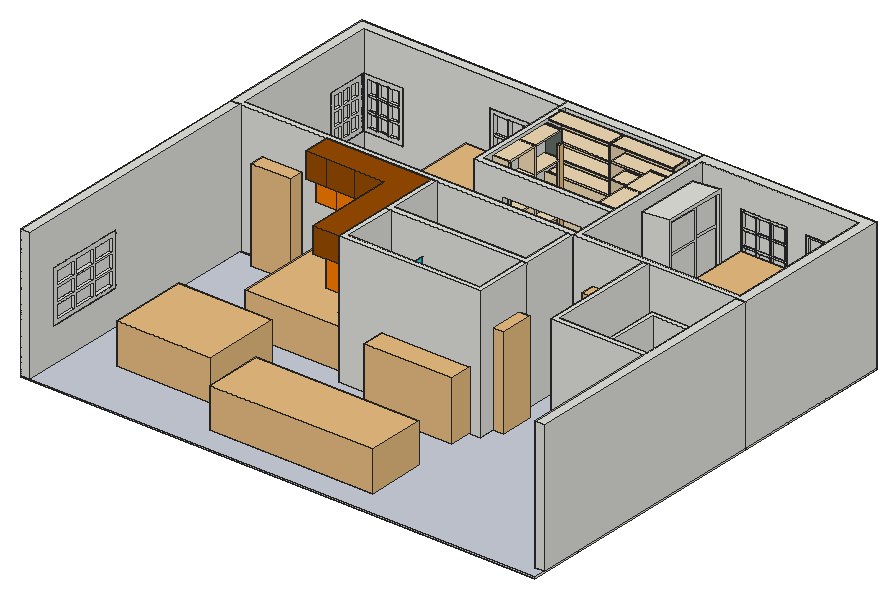
# SketchUp Ruby script. Lengths in inches.
U = 1.inch
M = Sketchup.active_model
def pt(a) = Geom::Point3d.new(a.map { |v| v * U })
def face(e, loops, mat)
  f = e.add_face(loops[0].map { |a| pt(a) })
  loops[1..].each { |l| e.add_face(l.map { |a| pt(a) }).erase! }
  f.material = f.back_material = mat if mat
  f
end
# faces: each face lists its corners as indices into pts; further lists are holes
def faces(e, pts, list, mat = nil) = list.each { |f| face(e, (f[0].is_a?(Array) ? f : [f]).map { |l| l.map { |i| pts[i] } }, mat) }
# xy, xz, yz: faces in a plane at the given z, y or x. An outline is a flat list of corners, or four numbers for a rectangle; further outlines are holes
def ring(l) = l.size == 4 ? [[l[0], l[1]], [l[2], l[1]], [l[2], l[3]], [l[0], l[3]]] : l.each_slice(2).to_a
def flat(e, list, mat, &to3) = list.each { |f| face(e, (f[0].is_a?(Array) ? f : [f]).map { |l| ring(l).map { |u, v| to3.(u, v) } }, mat) }
def xy(e, z, list, mat = nil) = flat(e, list, mat) { |x, y| [x, y, z] }
def xz(e, y, list, mat = nil) = flat(e, list, mat) { |x, z| [x, y, z] }
def yz(e, x, list, mat = nil) = flat(e, list, mat) { |y, z| [x, y, z] }
def lines(e, pts, list) = list.each { |a, b| e.add_line(pt(pts[a]), pt(pts[b])) }
# prism: a flat outline (further loops are holes) pulled along v
def prism(e, loops, v, mat = nil)
  f = face(e, loops, mat); d = Geom::Vector3d.new(v.map { |x| x * U })
  f.pushpull(f.normal.samedirection?(d) ? d.length : -d.length)
end
def box(e, o, s, mat = nil) = prism(e, [[o, [o[0] + s[0], o[1], o[2]], [o[0] + s[0], o[1] + s[1], o[2]], [o[0], o[1] + s[1], o[2]]]], [0, 0, s[2]], mat)
def at(x, y, z, deg = 0) = Geom::Transformation.translation(pt([x, y, z])) * Geom::Transformation.rotation(ORIGIN, Z_AXIS, deg.degrees)
def axes(o, x, y, z) = Geom::Transformation.new([*x, 0, *y, 0, *z, 0, *pt(o).to_a, 1])
def part(name) = M.definitions.add(name)
# library, detail: a bought-in or finely detailed component or shape, given as its bounding box
def library(name, o, s) = part(name).tap { |d| box(d.entities, o, s) }
def detail(e, o, s) = box(e.add_group.entities, o, s)
def put(e, d, t, mat = nil) = e.add_instance(d, t).tap { |i| i.material = mat if mat }
def group(e, t, mat = nil) = e.add_group.tap { |g| g.transformation = t; g.material = mat if mat }.entities
root = M.entities
M.materials.add("[Color C05]").color = [255, 127, 0]
M.materials.add("[Color C07]").color = [153, 76, 0]
M.materials.add("[Formica Laminate Light]").color = [242, 219, 181]
M.materials.add("[Marble Carrara Floor Tile]").color = [204, 208, 219]
M.materials.add("[Translucent Glass Tinted]").color = [8, 201, 241]
M.materials["[Translucent Glass Tinted]"].alpha = 0.48
M.materials.add("farrow and ball green smoke").color = [99, 111, 101]
c1 = library("Double bed ensemble",[0,-4.61,0],[113.04,95.21,114.59])
c2 = part("Group\#9")
yz(c2.entities,0,[[0,0,34.47,25.52]])
c3 = part("2 Panel Slidng Door Wardrobe")
g1 = group(c3.entities,at(68.39,-44.18,0,73.3))
g2 = group(g1,at(2.95,0.98,5.91))
g3 = group(g2,at(0,-32.89,0))
xy(g3,0,[[0,32.89,1.97,69.72]])
xy(g3,1.18,[[0,34.07,0.39,68.54]])
xy(g3,22.77,[[0,34.07,0.39,68.54]])
xy(g3,23.95,[[0,34.07,0.39,68.54]])
xy(g3,62.66,[[0,34.07,0.39,68.54]])
xy(g3,63.85,[[0,34.07,0.39,68.54]])
xy(g3,85.43,[[0,34.07,0.39,68.54]])
xy(g3,86.61,[[0,32.89,1.97,69.72]])
xz(g3,32.89,[[0,0,1.97,86.61]])
xz(g3,34.07,[[0,1.18,0.39,22.77],[0,23.95,0.39,62.66],[0,63.85,0.39,85.43]])
xz(g3,68.54,[[0,1.18,0.39,22.77],[0,23.95,0.39,62.66],[0,63.85,0.39,85.43]])
xz(g3,69.72,[[0,0,1.97,86.61]])
yz(g3,0,[[[32.89,0,69.72,86.61],[34.07,23.95,68.54,62.66],[34.07,1.18,68.54,22.77],[34.07,63.85,68.54,85.43]]])
yz(g3,0.39,[[34.07,1.18,68.54,22.77],[34.07,23.95,68.54,62.66],[34.07,63.85,68.54,85.43]])
yz(g3,1.97,[[32.89,0,69.72,86.61]])
put(g2,c2,axes([0.2,1.18,1.18],[1,0,0],[0,1,0],[0,0,0.84576]))
put(g2,c2,axes([0.2,1.18,63.85],[1,0,0],[0,1,0],[0,0,0.84576]))
g4 = group(g1,at(0.79,33.88,5.91))
g5 = group(g4,at(0,-32.89,0))
xy(g5,0,[[0,32.89,1.97,69.72]])
xy(g5,1.18,[[0,34.07,0.39,68.54]])
xy(g5,22.77,[[0,34.07,0.39,68.54]])
xy(g5,23.95,[[0,34.07,0.39,68.54]])
xy(g5,62.66,[[0,34.07,0.39,68.54]])
xy(g5,63.85,[[0,34.07,0.39,68.54]])
xy(g5,85.43,[[0,34.07,0.39,68.54]])
xy(g5,86.61,[[0,32.89,1.97,69.72]])
xz(g5,32.89,[[0,0,1.97,86.61]])
xz(g5,34.07,[[0,1.18,0.39,22.77],[0,23.95,0.39,62.66],[0,63.85,0.39,85.43]])
xz(g5,68.54,[[0,1.18,0.39,22.77],[0,23.95,0.39,62.66],[0,63.85,0.39,85.43]])
xz(g5,69.72,[[0,0,1.97,86.61]])
yz(g5,0,[[[32.89,0,69.72,86.61],[34.07,23.95,68.54,62.66],[34.07,1.18,68.54,22.77],[34.07,63.85,68.54,85.43]]])
yz(g5,0.39,[[34.07,1.18,68.54,22.77],[34.07,23.95,68.54,62.66],[34.07,63.85,68.54,85.43]])
yz(g5,1.97,[[32.89,0,69.72,86.61]])
put(g4,c2,axes([0.2,1.18,1.18],[1,0,0],[0,1,0],[0,0,0.84576]))
put(g4,c2,axes([0.2,1.18,63.85],[1,0,0],[0,1,0],[0,0,0.84576]))
g6 = group(g1,at(0,0,0))
xy(g6,0,[[0.98,0,23.62,71.69]])
xy(g6,3.9375,[[0,0,0.98,71.69]])
xy(g6,5.91,[[0,0.98,23.62,70.71]])
xy(g6,92.52,[[0,0.98,23.62,70.71]])
xy(g6,94.49,[[0,0,23.62,71.69]])
xz(g6,0,[[0.98,0,23.62,0,23.62,94.49,0,94.49,0,3.9375,0.98,3.9375]])
xz(g6,0.98,[[0,5.91,23.62,92.52]])
xz(g6,70.71,[[0,5.91,23.62,92.52]])
xz(g6,71.69,[[0.98,0,0.98,3.9375,0,3.9375,0,94.49,23.62,94.49,23.62,0]])
yz(g6,0,[[[0,3.9375,71.69,94.49],[0.98,5.91,70.71,92.52]]])
yz(g6,0.98,[[0,0,71.69,3.9375]])
yz(g6,23.62,[[[0,0,71.69,94.49],[0.98,5.91,70.71,92.52]],[0.98,5.91,70.71,92.52]])
c4 = library("Work Desk",[0,-12.98,-0.02],[78.74,36.6,34.67])
c5 = library("Coffee Table",[-15.75,-15.75,0],[31.5,31.5,16.93])
c6 = library("dining table",[-42.97,-35.1,0],[85.94,70.2,37.4])
c7 = library("Sofa-3(set)",[-65.09,-24.46,0],[149.34,77.78,36.35])
c8 = library("bathtub",[0,0,0],[65.51,30,28.53])
c9 = library("wc pot",[14.86,-58.21,0],[14.76,28.18,34.71])
c10 = library("Group\#110",[36.72,-0.92,0],[80.4,20.6,54.28])
c11 = part("tv unit")
p = [[0,0,0],[1,0,0],[1,1,0],[0,1700.8125,0],[1,1700.8125,0],[1,1701.8125,0]]
lines(c11.entities,p,[[0,1],[1,2],[2,0],[3,4],[5,3],[4,5]])
put(c11.entities,c10,at(2355.9375,1135.75,0))
c12 = library("Bathroom vanity ensemble",[0,0.5,0],[13.54,46.78,53.46])
c13 = library("clothes",[-0.07,-22.6875,1.29],[25.46,46.04,33.91])
c14 = library("Washing Machine 1",[-11.45,-11.86,0],[22.9,23.72,35.43])
c15 = part("Ktchen Unit Leg")
detail(c15.entities,[0,0,0],[1.97,1.97,3.9375])
c16 = library("skpE45D",[-24.47,-26.97,0],[48.94,53.94,77.79])
c17 = part("Group404\#1")
xy(c17.entities,0,[[-19,-20.8,-7.125,-7.72],[-5.9375,-20.8,5.9375,-7.72],[7.125,-20.8,19,-7.72],[-19,-6.54,-7.125,6.54],[-5.9375,-6.54,5.9375,6.54],
  [7.125,-6.54,19,6.54],[-19,7.72,-7.125,20.8],[-5.9375,7.72,5.9375,20.8],[7.125,7.72,19,20.8]])
c18 = part("Group403\#1")
prism(c18.entities,[[[21,-22.8,0],[-21,-22.8,0],[-21,22.8,0],[21,22.8,0]],[[-19,20.8,0],[-19,7.72,0],[-7.125,7.72,0],[-7.125,20.8,0]],[[-5.9375,20.8,0],[-5.9375,7.72,0],[5.9375,7.72,0],[5.9375,20.8,0]],[[19,20.8,0],[7.125,20.8,0],[7.125,7.72,0],[19,7.72,0]],[[-19,6.54,0],[-19,-6.54,0],[-7.125,-6.54,0],[-7.125,6.54,0]],[[-5.9375,-20.8,0],[5.9375,-20.8,0],[5.9375,-7.72,0],[-5.9375,-7.72,0]],[[-19,-20.8,0],[-7.125,-20.8,0],[-7.125,-7.72,0],[-19,-7.72,0]],[[-5.9375,-6.54,0],[5.9375,-6.54,0],[5.9375,6.54,0],[-5.9375,6.54,0]],[[19,-6.54,0],[19,6.54,0],[7.125,6.54,0],[7.125,-6.54,0]],[[19,-20.8,0],[19,-7.72,0],[7.125,-7.72,0],[7.125,-20.8,0]]],[0,0,3])
put(c18.entities,c17,at(0,0,1.5))
c19 = part("Group406\#1")
xy(c19.entities,0,[[-19,-20.8,-7.125,-7.72],[-5.9375,-20.8,5.9375,-7.72],[7.125,-20.8,19,-7.72],[-19,-6.54,-7.125,6.54],[-5.9375,-6.54,5.9375,6.54],
  [7.125,-6.54,19,6.54],[-19,7.72,-7.125,20.8],[-5.9375,7.72,5.9375,20.8],[7.125,7.72,19,20.8]])
c20 = part("Group405\#1")
prism(c20.entities,[[[-21,-22.8,0],[-21,22.8,0],[21,22.8,0],[21,-22.8,0]],[[-19,20.8,0],[-19,7.72,0],[-7.125,7.72,0],[-7.125,20.8,0]],[[-5.9375,20.8,0],[-5.9375,7.72,0],[5.9375,7.72,0],[5.9375,20.8,0]],[[7.125,20.8,0],[7.125,7.72,0],[19,7.72,0],[19,20.8,0]],[[19,-6.54,0],[19,6.54,0],[7.125,6.54,0],[7.125,-6.54,0]],[[-7.125,-20.8,0],[-7.125,-7.72,0],[-19,-7.72,0],[-19,-20.8,0]],[[5.9375,6.54,0],[-5.9375,6.54,0],[-5.9375,-6.54,0],[5.9375,-6.54,0]],[[-5.9375,-20.8,0],[5.9375,-20.8,0],[5.9375,-7.72,0],[-5.9375,-7.72,0]],[[19,-7.72,0],[7.125,-7.72,0],[7.125,-20.8,0],[19,-20.8,0]],[[-19,6.54,0],[-19,-6.54,0],[-7.125,-6.54,0],[-7.125,6.54,0]]],[0,0,3])
put(c20.entities,c19,at(0,0,1.5))
c21 = part("Group\#58")
box(c21.entities,[0,0,0],[48.98,0.75,78.74])
c22 = part("Group\#68")
box(c22.entities,[0,0,0],[23.39,19.69,0.75])
c23 = part("bau0015088853(v(70T310-05.02_ohne_Bohrungen))")
detail(c23.entities,[-12.16,-3.65,31.19],[22.02,7.3,13.75])
c24 = part("Group5\#2")
put(c24.entities,c23,at(0,0,0))
c25 = library("Group\#70",[0,22.05,7.17],[1.96,4.49,63.9])
c26 = library("Group\#72",[0,22.05,7.17],[1.96,4.49,63.9])
c27 = library("Group\#73",[0,19.81,7.17],[1.98,4.49,17.71])
c28 = part("Group\#63")
box(c28.entities,[0,0,0],[0.71,19.69,15.75])
c29 = part("Group\#51")
box(c29.entities,[-0.98,0,0],[47.48,19.69,0.75])
c30 = part("Group\#53")
box(c30.entities,[0,0,0.75],[0.75,19.69,77.99])
c31 = part("Group\#67")
box(c31.entities,[0,0,0],[23.39,19.69,0.75])
c32 = part("Group\#130")
box(c32.entities,[-0.24,0,0],[47.48,19.69,0.75])
c33 = part("Group\#54")
box(c33.entities,[0,0,0],[0.75,19.69,78.74])
c34 = part("Group\#56")
box(c34.entities,[0,0,0],[0.75,19.69,78.74])
c35 = library("Group\#128",[0,0,0],[36,17.91,84])
c36 = library("Group\#129",[0,0,0],[36,17.91,84])
c37 = library("Group\#132",[0,-0.01,0],[30,14.92,84])
c38 = library("Group\#134",[0,0,0],[14.93,30,84])
c39 = library("Group\#137",[0,0,0],[16.1,32.38,84])
c40 = part("Group431\#1")
xy(c40.entities,0,[[-20.0625,-26.0625,-7.48,-9.48],[-6.29,-26.0625,6.29,-9.48],[7.48,-26.0625,20.0625,-9.48],[-20.0625,-8.29,-7.48,8.29],[-6.29,-8.29,6.29,8.29],
  [7.48,-8.29,20.0625,8.29],[-20.0625,9.48,-7.48,26.0625],[-6.29,9.48,6.29,26.0625],[7.48,9.48,20.0625,26.0625]])
c41 = part("Group430\#1")
prism(c41.entities,[[[-24,30,0],[24,30,0],[24,-30,0],[-24,-30,0]],[[-7.48,-26.0625,0],[-7.48,-9.48,0],[-20.0625,-9.48,0],[-20.0625,-26.0625,0]],[[-6.29,9.48,0],[6.29,9.48,0],[6.29,26.0625,0],[-6.29,26.0625,0]],[[-20.0625,9.48,0],[-7.48,9.48,0],[-7.48,26.0625,0],[-20.0625,26.0625,0]],[[6.29,-26.0625,0],[6.29,-9.48,0],[-6.29,-9.48,0],[-6.29,-26.0625,0]],[[20.0625,-9.48,0],[7.48,-9.48,0],[7.48,-26.0625,0],[20.0625,-26.0625,0]],[[-20.0625,8.29,0],[-20.0625,-8.29,0],[-7.48,-8.29,0],[-7.48,8.29,0]],[[-6.29,8.29,0],[-6.29,-8.29,0],[6.29,-8.29,0],[6.29,8.29,0]],[[20.0625,-8.29,0],[20.0625,8.29,0],[7.48,8.29,0],[7.48,-8.29,0]],[[7.48,26.0625,0],[7.48,9.48,0],[20.0625,9.48,0],[20.0625,26.0625,0]]],[0,0,5.875])
put(c41.entities,c40,at(0,0,2.9375))
c42 = part("Group433\#1")
xy(c42.entities,0,[[-14.0625,-20.0625,-5.48,-7.48],[-4.29,-20.0625,4.29,-7.48],[5.48,-20.0625,14.0625,-7.48],[-14.0625,-6.29,-5.48,6.29],[-4.29,-6.29,4.29,6.29],
  [5.48,-6.29,14.0625,6.29],[-14.0625,7.48,-5.48,20.0625],[-4.29,7.48,4.29,20.0625],[5.48,7.48,14.0625,20.0625]])
c43 = part("Group432\#1")
prism(c43.entities,[[[-18,24,0],[18,24,0],[18,-24,0],[-18,-24,0]],[[-4.29,-20.0625,0],[4.29,-20.0625,0],[4.29,-7.48,0],[-4.29,-7.48,0]],[[4.29,-6.29,0],[4.29,6.29,0],[-4.29,6.29,0],[-4.29,-6.29,0]],[[14.0625,-6.29,0],[14.0625,6.29,0],[5.48,6.29,0],[5.48,-6.29,0]],[[-5.48,-20.0625,0],[-5.48,-7.48,0],[-14.0625,-7.48,0],[-14.0625,-20.0625,0]],[[-14.0625,6.29,0],[-14.0625,-6.29,0],[-5.48,-6.29,0],[-5.48,6.29,0]],[[14.0625,-7.48,0],[5.48,-7.48,0],[5.48,-20.0625,0],[14.0625,-20.0625,0]],[[-14.0625,20.0625,0],[-14.0625,7.48,0],[-5.48,7.48,0],[-5.48,20.0625,0]],[[-4.29,20.0625,0],[-4.29,7.48,0],[4.29,7.48,0],[4.29,20.0625,0]],[[5.48,20.0625,0],[5.48,7.48,0],[14.0625,7.48,0],[14.0625,20.0625,0]]],[0,0,5.875])
put(c43.entities,c42,at(0,0,2.9375))
c44 = part("Group435\#1")
xy(c44.entities,0,[[-14.0625,-20.0625,-5.48,-7.48],[-4.29,-20.0625,4.29,-7.48],[5.48,-20.0625,14.0625,-7.48],[-14.0625,-6.29,-5.48,6.29],[-4.29,-6.29,4.29,6.29],
  [5.48,-6.29,14.0625,6.29],[-14.0625,7.48,-5.48,20.0625],[-4.29,7.48,4.29,20.0625],[5.48,7.48,14.0625,20.0625]])
c45 = part("Group434\#1")
prism(c45.entities,[[[-18,24,0],[18,24,0],[18,-24,0],[-18,-24,0]],[[-14.0625,-20.0625,0],[-5.48,-20.0625,0],[-5.48,-7.48,0],[-14.0625,-7.48,0]],[[-4.29,-20.0625,0],[4.29,-20.0625,0],[4.29,-7.48,0],[-4.29,-7.48,0]],[[14.0625,-20.0625,0],[14.0625,-7.48,0],[5.48,-7.48,0],[5.48,-20.0625,0]],[[-14.0625,6.29,0],[-14.0625,-6.29,0],[-5.48,-6.29,0],[-5.48,6.29,0]],[[-4.29,6.29,0],[-4.29,-6.29,0],[4.29,-6.29,0],[4.29,6.29,0]],[[14.0625,-6.29,0],[14.0625,6.29,0],[5.48,6.29,0],[5.48,-6.29,0]],[[-5.48,20.0625,0],[-14.0625,20.0625,0],[-14.0625,7.48,0],[-5.48,7.48,0]],[[5.48,20.0625,0],[5.48,7.48,0],[14.0625,7.48,0],[14.0625,20.0625,0]],[[4.29,7.48,0],[4.29,20.0625,0],[-4.29,20.0625,0],[-4.29,7.48,0]]],[0,0,5.875])
put(c45.entities,c44,at(0,0,2.9375))
c46 = part("Group438\#1")
xy(c46.entities,0,[[-32.0625,-20.0625,-11.48,-7.48],[-10.29,-20.0625,10.29,-7.48],[11.48,-20.0625,32.0625,-7.48],[-32.0625,-6.29,-11.48,6.29],[-10.29,-6.29,10.29,6.29],
  [11.48,-6.29,32.0625,6.29],[-32.0625,7.48,-11.48,20.0625],[-10.29,7.48,10.29,20.0625],[11.48,7.48,32.0625,20.0625]])
c47 = part("Group437\#1")
prism(c47.entities,[[[36,24,0],[36,-24,0],[-36,-24,0],[-36,24,0]],[[11.48,-7.48,0],[11.48,-20.0625,0],[32.0625,-20.0625,0],[32.0625,-7.48,0]],[[10.29,-6.29,0],[10.29,6.29,0],[-10.29,6.29,0],[-10.29,-6.29,0]],[[32.0625,6.29,0],[11.48,6.29,0],[11.48,-6.29,0],[32.0625,-6.29,0]],[[-11.48,-6.29,0],[-11.48,6.29,0],[-32.0625,6.29,0],[-32.0625,-6.29,0]],[[11.48,20.0625,0],[11.48,7.48,0],[32.0625,7.48,0],[32.0625,20.0625,0]],[[-10.29,-7.48,0],[-10.29,-20.0625,0],[10.29,-20.0625,0],[10.29,-7.48,0]],[[-11.48,20.0625,0],[-32.0625,20.0625,0],[-32.0625,7.48,0],[-11.48,7.48,0]],[[-32.0625,-7.48,0],[-32.0625,-20.0625,0],[-11.48,-20.0625,0],[-11.48,-7.48,0]],[[10.29,20.0625,0],[-10.29,20.0625,0],[-10.29,7.48,0],[10.29,7.48,0]]],[0,0,5.875])
put(c47.entities,c46,at(0,0,2.9375))
p = [[355,382.125,48],[355,382.125,93.6],[397,382.125,93.6],[397,382.125,48],[415,382.125,48],[415,382.125,93.6],
  [457,382.125,93.6],[457,382.125,48],[297.97,348.05,79.88],[297.97,348.05,1.89],[107.125,217.125,120],[107.125,217.125,96.875],
  [132.96,217.125,120],[132.96,217.125,96.875],[160,196.68,120],[160,196.68,96.875],[160,176.125,120],[160,176.125,96.875],
  [160,155.92,120],[160,155.92,96.875],[106.77,229.125,72.875],[106.77,229.125,96.875],[130.02,229.125,72.875],[130.02,229.125,84.875],
  [130.02,229.125,96.875],[172,229.125,84.875],[172,201.83,72.875],[172,201.83,96.875],[172,168.03,72.875],[172,168.03,91.8125],
  [114.04,217.125,0],[114.04,217.125,36.125],[141.46,217.125,0],[141.46,217.125,36.125],[160,202.875,0],[160,202.875,34.1875],
  [160,182.37,0],[159.65,182.37,35.85],[160,163.58,0],[160,163.58,36.125],[172.64,382.125,96],[124.64,382.125,96],
  [124.64,382.125,36],[172.64,382.125,36],[9,382.125,36],[9,382.125,84],[45,382.125,84],[45,382.125,36],
  [9,380.28,84],[9,344.28,84],[9,344.28,36],[9,380.28,36],[9,98.14,79.78],[9,26.14,79.78],
  [9,26.14,31.78],[9,98.14,31.78]]
lines(root,p,[[0,1],[1,2],[2,3],[3,0],[4,5],[5,6],[6,7],[7,4],[8,9],[10,11],[12,13],[14,15],
  [16,17],[18,19],[20,21],[22,23],[23,24],[23,25],[26,27],[28,29],[30,31],[32,33],[34,35],[36,37],
  [38,39],[40,41],[41,42],[42,43],[43,40],[44,45],[45,46],[46,47],[47,44],[48,49],[49,50],[50,51],
  [51,48],[52,53],[53,54],[54,55],[55,52]])
put(root,c1,axes([440.65,373.67,0],[-0.72845,0,0],[0,-0.92053,0],[0,0,0.54258]))
put(root,c3,axes([323.05,305.125,0],[-0.27721,0.72908,0],[-0.93471,-0.3554,0],[0,0,1.18]))
put(root,c4,axes([439.38,292.77,0],[0,-0.44,0],[1,0,0],[0,0,0.8835]))
put(root,c5,at(71.7,288.55,3.42))
put(root,c6,at(88.65,88.9375,0))
put(root,c7,axes([267.9,23.82,25.4375],[-1,0,0],[0,-0.68,0],[0,0,1]))
put(root,c8,at(189,207.65,0))
put(root,c9,at(214.6,209.02,0))
put(root,c11,at(-2169.24,-1020.3,0))
put(root,c12,axes([297.26,163.86,0],[0,1.78351,0],[-1,0,0],[0,0,1.55]))
put(root,c13,at(386.14,209.17,41.68))
put(root,c14,axes([449.52,160.2,0],[1.17769,0,0],[0,1.36,0],[0,0,2.32]))
put(root,c15,axes([207.89,360.14,-3.9375],[0,1.23,0],[-0.78,0,0],[0,0,1]))
put(root,c15,axes([195.85,360.14,-3.9375],[0,1.23,0],[-0.78,0,0],[0,0,1]))
put(root,c15,axes([207.89,354.4,-3.9375],[0,1.23,0],[-0.78,0,0],[0,0,1]))
put(root,c15,axes([195.85,354.4,-3.9375],[0,1.23,0],[-0.78,0,0],[0,0,1]))
put(root,c15,axes([195.85,300.45,-3.9375],[0,1.23,0],[-0.78,0,0],[0,0,1]))
put(root,c15,axes([207.89,300.45,-3.9375],[0,1.23,0],[-0.78,0,0],[0,0,1]))
put(root,c15,axes([195.85,327.26,-3.9375],[0,1.23,0],[-0.78,0,0],[0,0,1]))
put(root,c15,axes([207.89,327.26,-3.9375],[0,1.23,0],[-0.78,0,0],[0,0,1]))
put(root,c16,axes([33.65,287.07,0],[-0.01471,0.40713,0],[-0.40713,-0.01471,0],[0,0,0.4074]))
put(root,c16,axes([46.02,321.09,0],[0.29762,0.27821,0],[-0.27821,0.29762,0],[0,0,0.4074]))
put(root,c1,axes([188.72,373.67,0],[-0.72845,0,0],[0,-0.92053,0],[0,0,0.54258]))
g7 = group(root,at(314,253.125,0))
xy(g7,0,[[0,-12,5,138],[125,-12,125,-7,149,-7,149,129,5,129,5,138,158,138,158,-12]])
xy(g7,48,[[41,129,83,138],[101,129,143,138]])
xy(g7,84,[[18,-12,54,-7]])
xy(g7,93.6,[[41,129,83,138],[101,129,143,138]])
xy(g7,120,[[[0,-12,158,138],[5,-7,149,129]]])
xz(g7,-12,[[0,0,18,0,18,84,54,84,54,0,158,0,158,120,0,120]])
xz(g7,-7,[[5,0,18,0,18,84,54,84,54,0,149,0,149,120,5,120]])
xz(g7,129,[[[5,0,149,120],[41,48,83,93.6],[101,48,143,93.6]]])
xz(g7,138,[[[0,0,158,120],[41,48,83,93.6],[101,48,143,93.6]]])
yz(g7,0,[[-12,0,138,120]])
yz(g7,5,[[-7,0,129,120]])
yz(g7,18,[[-12,0,-7,84]])
yz(g7,41,[[129,48,138,93.6]])
yz(g7,54,[[-12,0,-7,84]])
yz(g7,83,[[129,48,138,93.6]])
yz(g7,101,[[129,48,138,93.6]])
yz(g7,143,[[129,48,138,93.6]])
yz(g7,149,[[-7,0,129,120]])
yz(g7,158,[[-12,0,138,120]])
p = [[18,-7,0],[54,-7,0]]
lines(g7,p,[[0,1]])
put(root,c18,axes([376,385.125,70.8],[1,0,0],[0,0,1],[0,-1,0]))
put(root,c20,axes([436,385.125,70.8],[1,0,0],[0,0,1],[0,-1,0]))
g8 = group(root,at(250.36,361.79,7.4),"[Formica Laminate Light]")
box(g8,[0,0,1.07],[1.8,15.56,111.53])
g9 = group(root,at(194.57,361.79,118.93),"[Formica Laminate Light]")
box(g9,[-0.57,0,0],[114.53,15.56,1.07])
g10 = group(root,at(308.53,361.79,7.4),"[Formica Laminate Light]")
box(g10,[0,0,0],[1.8,15.56,112.6])
put(root,c21,axes([192.2,377.36,7.4],[2.41209,0,0],[0,0.79068,0],[0,0,1.43]),"[Formica Laminate Light]")
g11 = group(root,at(196.375,361.79,7.4),"[Formica Laminate Light]")
box(g11,[-2.375,0,0],[114.52,15.56,1.07])
put(root,c22,axes([252.17,361.79,90.33],[2.41209,0,0],[0,0.79068,0],[0,0,1.43]),"[Formica Laminate Light]")
put(root,c22,axes([252.17,361.79,104.63],[2.41209,0,0],[0,0.79068,0],[0,0,1.43]),"[Formica Laminate Light]")
put(root,c22,axes([194,361.79,76.03],[2.41209,0,0],[0,0.79068,0],[0,0,1.43]),"[Formica Laminate Light]")
put(root,c22,axes([194,361.79,90.33],[2.41209,0,0],[0,0.79068,0],[0,0,1.43]),"[Formica Laminate Light]")
put(root,c22,axes([194,361.79,104.63],[2.41209,0,0],[0,0.79068,0],[0,0,1.43]),"[Formica Laminate Light]")
put(root,c22,axes([252.17,361.79,76.03],[2.41209,0,0],[0,0.79068,0],[0,0,1.43]),"[Formica Laminate Light]")
put(root,c24,axes([209.69,354.53,8.29],[-0.03071,0,0],[0,0,0.03937],[0,0.04843,0]))
put(root,c24,axes([209.69,354.53,23.68],[-0.03071,0,0],[0,0,0.03937],[0,0.04843,0]))
put(root,c24,axes([209.69,354.53,39.35],[-0.03071,0,0],[0,0,0.03937],[0,0.04843,0]))
put(root,c24,axes([209.69,354.53,69.875],[-0.03071,0,0],[0,0,0.03937],[0,0.04843,0]))
put(root,c24,axes([209.69,354.53,54.28],[-0.03071,0,0],[0,0,0.03937],[0,0.04843,0]))
put(root,c25,axes([227.71,355.78,0],[0,1.23,0],[-0.78,0,0],[0,0,1.5]))
put(root,c26,axes([227.71,298.76,0],[0,1.23,0],[-0.78,0,0],[0,0,1]))
put(root,c27,axes([225.96,358.97,0],[0,1.23,0],[-0.78,0,0],[0,0,1]))
g12 = group(root,at(209.19,358.61,0),"[Formica Laminate Light]")
box(g12,[-15.35,0,0],[15.35,0.92,31.5])
put(root,c28,axes([209.19,358.66,31.5],[0,1.23,0],[-0.78,0,0],[0,0,1]),"farrow and ball green smoke")
put(root,c21,axes([193.84,298.37,0],[0,1.23,0],[-0.78,0,0],[0,0,1]),"[Formica Laminate Light]")
put(root,c22,axes([209.19,328.95,15.59],[0,1.23,0],[-0.78,0,0],[0,0,1]),"[Formica Laminate Light]")
put(root,c29,axes([209.19,300.5,0],[0,1.23,0],[-0.78,0,0],[0,0,1.5]),"[Formica Laminate Light]")
put(root,c28,axes([209.19,358.66,47.24],[0,1.23,0],[-0.78,0,0],[0,0,1]),"farrow and ball green smoke")
put(root,c30,axes([209.19,328.03,0],[0,1.23,0],[-0.78,0,0],[0,0,1.5]),"[Formica Laminate Light]")
put(root,c22,axes([209.19,299.29,23.39],[0,1.23,0],[-0.78,0,0],[0,0,1.5]),"[Formica Laminate Light]")
put(root,c31,axes([209.19,299.29,93.54],[0,1.23,0],[-0.78,0,0],[0,0,1.5]),"[Formica Laminate Light]")
put(root,c28,axes([209.19,358.66,94.49],[0,1.23,0],[-0.78,0,0],[0,0,1.5]),"farrow and ball green smoke")
put(root,c32,axes([209.19,299.58,116.99],[0,1.23,0],[-0.78,0,0],[0,0,1.5]),"[Formica Laminate Light]")
put(root,c33,axes([209.19,298.37,0],[0,1.23,0],[-0.78,0,0],[0,0,1.5]),"[Formica Laminate Light]")
put(root,c22,axes([209.19,328.95,46.77],[0,1.23,0],[-0.78,0,0],[0,0,1.5]),"[Formica Laminate Light]")
put(root,c22,axes([209.19,328.95,70.16],[0,1.23,0],[-0.78,0,0],[0,0,1.5]),"[Formica Laminate Light]")
put(root,c34,axes([209.19,357.69,0],[0,1.23,0],[-0.78,0,0],[0,0,1]),"[Formica Laminate Light]")
put(root,c22,axes([209.19,299.29,70.16],[0,1.23,0],[-0.78,0,0],[0,0,1.5]),"[Formica Laminate Light]")
put(root,c22,axes([209.19,299.29,46.77],[0,1.23,0],[-0.78,0,0],[0,0,1.5]),"[Formica Laminate Light]")
put(root,c22,axes([209.19,328.95,93.54],[0,1.23,0],[-0.78,0,0],[0,0,1.5]),"[Formica Laminate Light]")
put(root,c22,axes([298.65,319.31,17.48],[0,1.23,0],[0.78,0,0],[0,0,1]),"[Formica Laminate Light]")
put(root,c29,axes([298.65,290.86,1.89],[0,1.23,0],[0.78,0,0],[0,0,1.5]),"[Formica Laminate Light]")
put(root,c28,axes([298.65,349.02,49.13],[0,1.23,0],[0.78,0,0],[0,0,1]),"farrow and ball green smoke")
put(root,c30,axes([298.65,318.39,1.89],[0,1.23,0],[0.78,0,0],[0,0,1.5]),"[Formica Laminate Light]")
put(root,c22,axes([298.65,289.65,25.28],[0,1.23,0],[0.78,0,0],[0,0,1.5]),"[Formica Laminate Light]")
put(root,c31,axes([298.65,289.65,95.43],[0,1.23,0],[0.78,0,0],[0,0,1.5]),"[Formica Laminate Light]")
put(root,c28,axes([298.65,349.02,96.38],[0,1.23,0],[0.78,0,0],[0,0,1.5]),"farrow and ball green smoke")
put(root,c32,axes([298.65,289.9375,118.88],[0,1.23,0],[0.78,0,0],[0,0,1.5]),"[Formica Laminate Light]")
put(root,c33,axes([298.65,288.73,1.89],[0,1.23,0],[0.78,0,0],[0,0,1.5]),"[Formica Laminate Light]")
put(root,c22,axes([298.65,319.31,48.66],[0,1.23,0],[0.78,0,0],[0,0,1.5]),"[Formica Laminate Light]")
put(root,c22,axes([298.65,319.31,72.05],[0,1.23,0],[0.78,0,0],[0,0,1.5]),"[Formica Laminate Light]")
put(root,c34,axes([298.65,348.05,1.89],[0,1.23,0],[0.78,0,0],[0,0,1]),"[Formica Laminate Light]")
put(root,c22,axes([298.65,289.65,72.05],[0,1.23,0],[0.78,0,0],[0,0,1.5]),"[Formica Laminate Light]")
put(root,c22,axes([298.65,289.65,48.66],[0,1.23,0],[0.78,0,0],[0,0,1.5]),"[Formica Laminate Light]")
put(root,c22,axes([298.65,319.31,95.43],[0,1.23,0],[0.78,0,0],[0,0,1.5]),"[Formica Laminate Light]")
g13 = group(root,at(185,283.73,0))
xy(g13,0,[[4,0,30,5],[102,0,129,5],[4,5,4,107.4,129,107.4,129,98.4,9,98.4,9,5]])
xy(g13,97.89,[[30,0,102,5]])
xy(g13,120,[[4,0,129,0,129,5,9,5,9,98.4,129,98.4,129,107.4,4,107.4]])
xz(g13,0,[[4,0,30,0,30,97.89,102,97.89,102,0,129,0,129,120,4,120]])
xz(g13,5,[[9,0,9,120,129,120,129,0,102,0,102,97.89,30,97.89,30,0]])
xz(g13,98.4,[[9,0,129,120]])
xz(g13,107.4,[[4,0,129,120]])
yz(g13,4,[[0,0,107.4,120]])
yz(g13,9,[[5,0,98.4,120]])
yz(g13,30,[[0,0,5,97.89]])
yz(g13,102,[[0,0,5,97.89]])
yz(g13,129,[[0,0,5,120],[98.4,0,107.4,120]])
g14 = group(root,at(0,241.125,0))
xy(g14,0,[[0,0,29.1875,5],[65.1875,0,271.68,5],[301.68,0,314,5]])
xy(g14,36,[[0,103.16,9,139.16],[9,141,45,150],[124.64,141,172.64,150]])
xy(g14,84,[[29.1875,0,65.1875,5],[271.68,0,301.68,5],[0,103.16,9,139.16],[9,141,45,150]])
xy(g14,96,[[124.64,141,172.64,150]])
xy(g14,120,[[0,0,314,0,314,5,9,5,9,141,189,141,189,150,0,150]])
xz(g14,0,[[0,0,29.1875,0,29.1875,84,65.1875,84,65.1875,0,271.68,0,271.68,84,301.68,84,301.68,0,314,0,314,120,0,120]])
xz(g14,5,[[9,0,9,120,314,120,314,0,301.68,0,301.68,84,271.68,84,271.68,0,65.1875,0,65.1875,84,29.1875,84,29.1875,0]])
xz(g14,103.16,[[0,36,9,84]])
xz(g14,139.16,[[0,36,9,84]])
xz(g14,141,[[[9,0,189,0,189,120,9,120,9,84,45,84,45,36,9,36],[124.64,36,172.64,96]]])
xz(g14,150,[[[0,0,189,120],[124.64,36,172.64,96],[9,36,45,84]]])
yz(g14,0,[[0,0,5,120],[[5,0,150,120],[103.16,36,139.16,84]]])
yz(g14,9,[[[5,0,141,0,141,36,150,36,150,84,141,84,141,120,5,120],[103.16,36,139.16,84]]])
yz(g14,29.1875,[[0,0,5,84]])
yz(g14,45,[[141,36,150,84]])
yz(g14,65.1875,[[0,0,5,84]])
yz(g14,124.64,[[141,36,150,96]])
yz(g14,172.64,[[141,36,150,96]])
yz(g14,189,[[141,0,150,120]])
yz(g14,271.68,[[0,0,5,84]])
yz(g14,301.68,[[0,0,5,84]])
yz(g14,314,[[0,0,5,120]])
put(root,c35,at(29.1875,228.21,0))
put(root,c36,at(332,228.21,0))
g15 = group(root,at(184,135.125,0))
xy(g15,0,[[0,53,5,106],[5,53,125,58],[125,53,130,106]])
xy(g15,120,[[0,53,130,53,130,106,125,106,125,58,5,58,5,106,0,106]])
xz(g15,53,[[0,0,130,120]])
xz(g15,58,[[5,0,125,120]])
xz(g15,106,[[0,0,5,120],[125,0,130,120]])
yz(g15,0,[[53,0,106,120]])
yz(g15,5,[[58,0,106,120]])
yz(g15,125,[[58,0,106,120]])
yz(g15,130,[[53,0,106,120]])
p = [[130,53,0],[130,0,0]]
lines(g15,p,[[0,1]])
put(root,c37,at(271.68,231.21,0))
g16 = group(root,at(184,135.125,0))
xy(g16,0,[[33.41,5,34.6,53],[125,13.82,130,43.82]])
xy(g16,84,[[125,13.82,130,43.82]])
xy(g16,91.3125,[[33.41,5,34.6,53]])
xy(g16,120,[[0,0,130,0,130,53,125,53,125,5,5,5,5,53,0,53]])
xz(g16,0,[[0,0,130,120]])
xz(g16,5,[[5,0,33.41,120],[33.41,0,34.6,91.3125],[34.6,0,125,120],[33.41,91.3125,34.6,120]])
xz(g16,13.82,[[125,0,130,84]])
xz(g16,43.82,[[125,0,130,84]])
xz(g16,53,[[0,0,5,120],[33.41,0,34.6,91.3125],[125,0,130,120]])
yz(g16,0,[[0,0,53,120]])
yz(g16,5,[[5,0,53,120]])
yz(g16,33.41,[[5,0,53,91.3125]],"[Translucent Glass Tinted]")
yz(g16,34.6,[[5,0,53,91.3125]],"[Translucent Glass Tinted]")
yz(g16,125,[[5,0,5,120,53,120,53,0,43.82,0,43.82,84,13.82,84,13.82,0]])
yz(g16,130,[[0,0,13.82,0,13.82,84,43.82,84,43.82,0,53,0,53,120,0,120]])
put(root,c38,at(309,148.94,0))
g17 = group(root,at(378,11.1875,0))
xy(g17,0,[[85,0,94,40.9375],[0,123.9375,5,140.84],[5,123.9375,85,128.9375],[0,173.22,5,229.9375]])
xy(g17,84,[[0,140.84,5,173.22]])
xy(g17,120,[[85,0,94,229.9375],[0,123.9375,85,123.9375,85,128.9375,5,128.9375,5,229.9375,0,229.9375]])
xz(g17,0,[[85,0,94,120]])
xz(g17,123.9375,[[0,0,85,120]])
xz(g17,128.9375,[[5,0,85,120]])
xz(g17,140.84,[[0,0,5,84]])
xz(g17,173.22,[[0,0,5,84]])
xz(g17,229.9375,[[0,0,5,120],[85,0,94,120]])
yz(g17,0,[[123.9375,0,123.9375,120,229.9375,120,229.9375,0,173.22,0,173.22,84,140.84,84,140.84,0]])
yz(g17,5,[[128.9375,0,140.84,0,140.84,84,173.22,84,173.22,0,229.9375,0,229.9375,120,128.9375,120]])
yz(g17,85,[[0,0,123.9375,120],[128.9375,0,229.9375,120]])
yz(g17,94,[[0,0,229.9375,120]])
g18 = group(root,at(88.04,135.125,12.875),"[Color C05]")
xy(g18,60,[[83.96,0,95.96,94],[0,94,95.96,106]])
xy(g18,84,[[83.96,0,95.96,0,95.96,106,0,106,0,94,83.96,94]])
xz(g18,0,[[83.96,60,95.96,84]])
xz(g18,94,[[0,60,83.96,84]])
xz(g18,106,[[0,60,95.96,84]])
yz(g18,0,[[94,60,106,84]])
yz(g18,83.96,[[0,60,94,84]])
yz(g18,95.96,[[0,60,94,84],[94,60,106,84]])
g19 = group(root,at(88.04,135.125,96.875),"[Color C07]")
xy(g19,0,[[71.96,0,95.96,82],[0,82,95.96,106]])
xy(g19,23.125,[[71.96,0,95.96,0,95.96,106,0,106,0,82,71.96,82]])
xz(g19,0,[[71.96,0,95.96,23.125]])
xz(g19,82,[[0,0,71.96,23.125]])
xz(g19,106,[[0,0,95.96,23.125]])
yz(g19,0,[[82,0,106,23.125]])
yz(g19,71.96,[[0,0,82,23.125]])
yz(g19,95.96,[[82,0,106,23.125]])
g20 = group(root,at(88.04,147.62,0))
detail(g20,[0,0,0],[95.96,93.51,36])
put(root,c39,at(378,152.03,0))
put(root,c41,axes([148.64,388,66],[1,0,0],[0,0,1],[0,-1,0]))
put(root,c43,axes([27,388,60],[1,0,0],[0,0,1],[0,-1,0]))
put(root,c45,axes([3.125,362.28,60],[0,1,0],[0,0,1],[1,0,0]))
g21 = group(root,at(0,0,-1))
xy(g21,0,[[[0,0,472,241.125],[428.11,140.125,432.11,140.125,432.11,184.4375,463,184.4375,463,188.4375,428.11,188.4375]],[[0,241.125,472,391.125],[209.19,297.0625,209.87,299.29],[209.19,357.69,209.87,359.53]]],"[Marble Carrara Floor Tile]")
xy(g21,1,[[0,0,9,241.125],[428.11,140.125,428.11,188.4375,463,188.4375,463,184.4375,432.11,184.4375,432.11,140.125]])
xy(g21,1,[[209.19,297.0625,209.87,299.29],[209.19,357.69,209.87,359.53]],"farrow and ball green smoke")
xy(g21,32.78,[[0,26.14,9,98.14]])
xy(g21,80.78,[[0,26.14,9,98.14]])
xy(g21,121,[[0,0,9,241.125],[428.11,140.125,432.11,140.125,432.11,184.4375,463,184.4375,463,188.4375,428.11,188.4375]])
xz(g21,0,[[0,0,472,1],[0,1,9,121]])
xz(g21,26.14,[[0,32.78,9,80.78]])
xz(g21,98.14,[[0,32.78,9,80.78]])
xz(g21,140.125,[[428.11,0,432.11,1],[428.11,1,432.11,121]])
xz(g21,184.4375,[[432.11,0,463,1],[432.11,1,463,121]])
xz(g21,188.4375,[[428.11,0,463,1],[428.11,1,463,121]])
xz(g21,241.125,[[0,1,9,121]])
xz(g21,297.0625,[[209.19,0,209.87,1]])
xz(g21,299.29,[[209.19,0,209.87,1]])
xz(g21,299.29,[[209.19,1,209.19,78.99,209.87,117.99,209.87,1]],"farrow and ball green smoke")
xz(g21,357.69,[[209.19,0,209.87,1]])
xz(g21,357.69,[[209.19,1,209.87,78.99]],"farrow and ball green smoke")
xz(g21,359.53,[[209.19,0,209.87,1],[209.19,47.5,209.87,48.99]])
xz(g21,359.53,[[209.19,1,209.87,31.75],[209.19,33.24,209.87,47.5],[209.19,48.99,209.87,63.24],[209.19,64.74,209.87,78.99]],"farrow and ball green smoke")
xz(g21,391.125,[[0,0,472,1]])
yz(g21,0,[[0,0,241.125,1],[241.125,0,391.125,1],[[0,1,241.125,121],[26.14,32.78,98.14,80.78]]])
yz(g21,9,[[[0,1,241.125,121],[26.14,32.78,98.14,80.78]]])
yz(g21,209.19,[[297.0625,0,299.29,1],[357.69,0,359.53,1]])
yz(g21,209.87,[[297.0625,0,299.29,1],[357.69,0,359.53,1]])
yz(g21,209.87,[[357.69,1,359.53,83.68],[359.53,31.75,359.55,33.24],[359.53,47.5,359.55,48.99],[359.53,63.24,359.55,64.74],[359.53,78.99,359.55,83.68],
  [299.29,83.68,299.29,117.99,299.31,117.97],[299.31,117.97,299.29,117.99,299.31,117.99]],"farrow and ball green smoke")
yz(g21,428.11,[[140.125,0,188.4375,1],[140.125,1,188.4375,121]])
yz(g21,432.11,[[140.125,0,184.4375,1],[140.125,1,184.4375,121]])
yz(g21,463,[[184.4375,0,188.4375,1],[184.4375,1,188.4375,121]])
yz(g21,472,[[0,0,241.125,1],[241.125,0,391.125,1]])
put(root,c47,axes([3.125,62.14,55.78],[0,1,0],[0,0,1],[1,0,0]))
